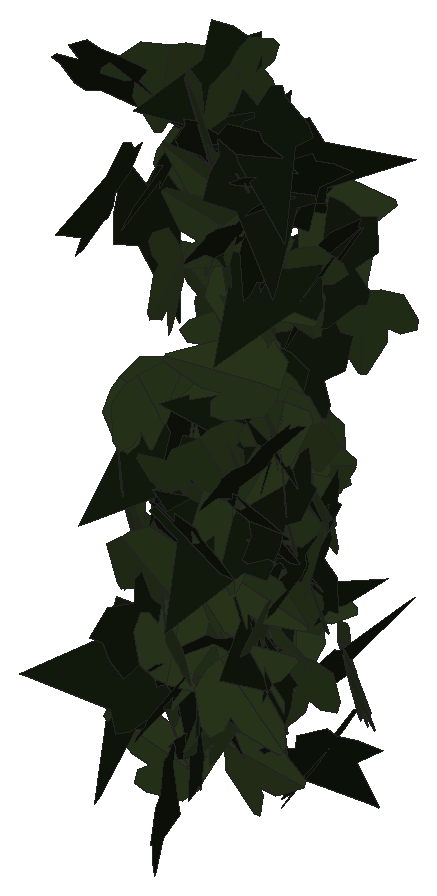
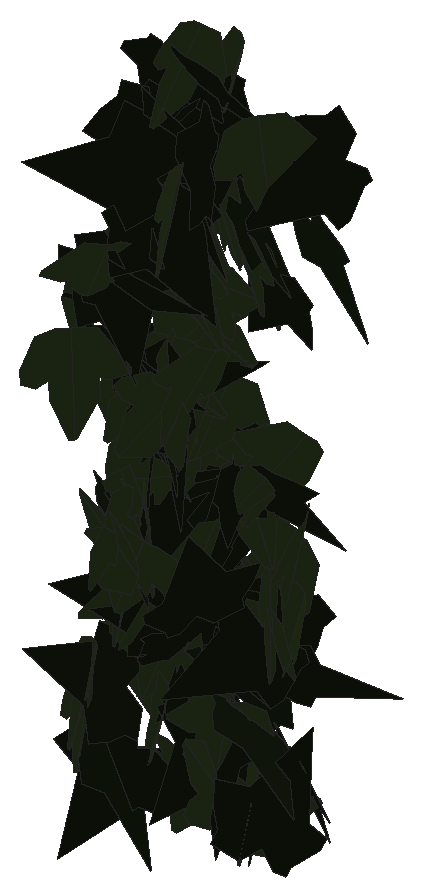
# SketchUp Ruby script. Lengths in inches.
U = 1.inch
M = Sketchup.active_model
def pt(a) = Geom::Point3d.new(a.map { |v| v * U })
def face(e, loops, mat)
  f = e.add_face(loops[0].map { |a| pt(a) })
  loops[1..].each { |l| e.add_face(l.map { |a| pt(a) }).erase! }
  f.material = f.back_material = mat if mat
  f
end
# faces: each face lists its corners as indices into pts; further lists are holes
def faces(e, pts, list, mat = nil) = list.each { |f| face(e, (f[0].is_a?(Array) ? f : [f]).map { |l| l.map { |i| pts[i] } }, mat) }
# xy, xz, yz: faces in a plane at the given z, y or x. An outline is a flat list of corners, or four numbers for a rectangle; further outlines are holes
def ring(l) = l.size == 4 ? [[l[0], l[1]], [l[2], l[1]], [l[2], l[3]], [l[0], l[3]]] : l.each_slice(2).to_a
def flat(e, list, mat, &to3) = list.each { |f| face(e, (f[0].is_a?(Array) ? f : [f]).map { |l| ring(l).map { |u, v| to3.(u, v) } }, mat) }
def xy(e, z, list, mat = nil) = flat(e, list, mat) { |x, y| [x, y, z] }
def xz(e, y, list, mat = nil) = flat(e, list, mat) { |x, z| [x, y, z] }
def yz(e, x, list, mat = nil) = flat(e, list, mat) { |y, z| [x, y, z] }
def lines(e, pts, list) = list.each { |a, b| e.add_line(pt(pts[a]), pt(pts[b])) }
# prism: a flat outline (further loops are holes) pulled along v
def prism(e, loops, v, mat = nil)
  f = face(e, loops, mat); d = Geom::Vector3d.new(v.map { |x| x * U })
  f.pushpull(f.normal.samedirection?(d) ? d.length : -d.length)
end
def box(e, o, s, mat = nil) = prism(e, [[o, [o[0] + s[0], o[1], o[2]], [o[0] + s[0], o[1] + s[1], o[2]], [o[0], o[1] + s[1], o[2]]]], [0, 0, s[2]], mat)
def at(x, y, z, deg = 0) = Geom::Transformation.translation(pt([x, y, z])) * Geom::Transformation.rotation(ORIGIN, Z_AXIS, deg.degrees)
def axes(o, x, y, z) = Geom::Transformation.new([*x, 0, *y, 0, *z, 0, *pt(o).to_a, 1])
def part(name) = M.definitions.add(name)
# library, detail: a bought-in or finely detailed component or shape, given as its bounding box
def library(name, o, s) = part(name).tap { |d| box(d.entities, o, s) }
def detail(e, o, s) = box(e.add_group.entities, o, s)
def put(e, d, t, mat = nil) = e.add_instance(d, t).tap { |i| i.material = mat if mat }
def group(e, t, mat = nil) = e.add_group.tap { |g| g.transformation = t; g.material = mat if mat }.entities
root = M.entities
M.materials.add("efeu1").color = [18, 25, 13]
M.materials.add("efeu2").color = [43, 57, 29]
c1 = part("ivyleaf_9")
p = [[1.54,2.16,1.25],[1.36,2.04,1.19],[-0.21,0.99,0.68],[-0.71,1.11,0.82],[-0.85,0.86,0.67],[-0.8,0.17,0.21],
  [-0.9,-0.01,0.1],[-0.67,-0.16,-0.02],[-0.08,-0.08,-0.05],[-0.03,-0.6,-0.4],[0.65,-0.88,-0.66],[0.83,-0.6,-0.49],
  [1.29,-0.42,-0.43],[1.8125,-0.07,-0.26],[1.21,0.44,0.15]]
faces(c1.entities,p,[[0,1,2,3,4,5,6,7,8,9,10,11,12,13,14]],"efeu1")
c2 = part("ivyleaf_10")
p = [[0,0.5,-0.03],[-0.0625,2.02,-0.43],[-0.19,2.01,-0.46],[-0.54,1.05,-0.29],[-0.52,0.625,-0.18],[-0.83,0.76,-0.28],
  [-1.16,0.64,-0.33],[-1.15,0.33,-0.24],[-0.77,-0.39,0.02],[-0.3,-0.51,0.16],[0.04,-0.48,0.23],[-0.02,2.01,-0.4375],
  [-0.06,2.01,-0.43],[0.04,-0.49,0.23],[0.67,-0.49,0.14],[1.38,0.36,-0.2],[1.375,0.51,-0.24],[0.81,0.65,-0.19],
  [0.62,0.59,-0.15],[0.6,1.09,-0.28],[0.5,1.23,-0.31]]
faces(c2.entities,p,[[0,1,2,3,4,5,6,7,8,9,10],[11,12,0,13,14,15,16,17,18,19,20]],"efeu2")
put(root,c1,axes([50.09,225.1875,214.06],[0.37177,-0.08571,0.32318],[-0.31461,0.07392,0.38152],[-0.11318,-0.48702,0.00103]))
put(root,c1,axes([49.87,224.07,222.45],[0.4848,0.06359,0.10454],[0.10369,0.01327,-0.48895],[-0.06496,0.49576,-0.00032]))
put(root,c2,axes([50.18,224.51,216.72],[-0.36902,0.33646,-0.02481],[0.00916,-0.02676,-0.4992],[-0.33725,-0.36889,0.01359]))
put(root,c1,axes([50.28,224.42,214.78],[-0.4013,0.06407,-0.29129],[0.2902,-0.02882,-0.40614],[-0.06883,-0.49504,-0.01405]))
put(root,c1,axes([50.54,223.71,221.2],[-0.31294,0.386,0.05546],[-0.02705,0.04945,-0.49681],[-0.38902,-0.31394,-0.01007]))
put(root,c2,axes([50.24,224.37,217.61],[-0.16912,0.46737,-0.05444],[0.00672,-0.05544,-0.49687],[-0.47048,-0.1688,0.01247]))
put(root,c1,axes([50.63,224.73,215.2],[-0.14528,0.43672,0.19536],[-0.19015,0.13464,-0.4424],[-0.43902,-0.20284,0.12697]))
put(root,c1,axes([50.5,225.86,217.19],[-0.28944,-0.24669,0.3246],[0.25134,0.20548,0.38027],[-0.32102,0.3833,0.00506]))
put(root,c2,axes([50.5,224.59,216.43],[-0.46152,0.18451,-0.05441],[-0.02286,-0.19302,-0.46067],[-0.191,-0.42273,0.1866]))
put(root,c2,axes([50.6,224.37,216.77],[0.08705,-0.42674,-0.24559],[-0.05203,0.24003,-0.43552],[0.48961,0.10138,-0.00261]))
put(root,c2,axes([50.85,224.59,213.82],[0.20562,0.14332,0.43264],[-0.37231,-0.22095,0.25014],[0.26288,-0.42502,0.01585]))
put(root,c1,axes([50.99,223.83,215.36],[-0.35853,0.0255,0.34757],[-0.34841,-0.03802,-0.3566],[0.00824,-0.4979,0.04503]))
put(root,c2,axes([50.72,224.45,222.61],[-0.33487,-0.36606,0.06215],[-0.03843,-0.04907,-0.4961],[0.36931,-0.33703,0.00473]))
put(root,c2,axes([50.78,224.49,214.39],[-0.32227,0.31708,0.21355],[-0.15272,0.14927,-0.4521],[-0.35046,-0.35662,0.00063]))
put(root,c2,axes([50.53,224.15,218.53],[0.15002,0.32465,0.34942],[0.10753,0.33385,-0.35635],[-0.46468,0.18207,0.03034]))
put(root,c1,axes([50.85,224.58,221.72],[-0.36486,0.27484,-0.20332],[0.15828,-0.12777,-0.45675],[-0.30302,-0.39767,0.00623]))
put(root,c1,axes([50.49,224.41,220.9],[-0.21631,-0.07779,-0.44403],[0.42341,0.13397,-0.22973],[0.15471,-0.4754,0.00792]))
put(root,c1,axes([50.45,224.5,216.25],[0.43193,0.14293,0.20739],[0.18332,0.10392,-0.45342],[-0.17272,0.46773,0.03737]))
put(root,c1,axes([50.95,224.33,218.04],[-0.48296,-0.11685,0.05568],[-0.05363,-0.0151,-0.49689],[0.1178,-0.48592,0.00205]))
put(root,c2,axes([50.66,224.18,218.52],[0.2277,0.3873,0.21943],[0.03568,0.2298,-0.44263],[-0.44371,0.21723,0.07701]))
put(root,c2,axes([50.84,224.61,221.35],[0.42787,-0.2583,0.01446],[0.01413,-0.00456,-0.49978],[0.25831,0.42809,0.00339]))
put(root,c1,axes([51.09,224.625,214.91],[0.288,0.05961,-0.40436],[-0.40809,0.01432,-0.28854],[-0.02282,0.49623,0.0569]))
put(root,c1,axes([50.96,224.62,218.37],[-0.13753,0.12973,-0.46288],[0.34145,-0.31253,-0.18904],[-0.33837,-0.3681,-0.00263]))
put(root,c2,axes([50.93,224.76,215.2],[0.43155,0.23257,0.09838],[0.04569,0.11966,-0.48332],[-0.24835,0.42614,0.08203]))
put(root,c1,axes([50.92,223.7,216.22],[0.00971,-0.04193,-0.49814],[-0.02923,0.49734,-0.04244],[0.49905,0.02994,0.00721]))
put(root,c2,axes([51.05,224.84,214.23],[0.15991,-0.41773,0.22346],[-0.08225,0.20778,0.44728],[-0.46654,-0.17981,-0.00227]))
put(root,c2,axes([50.92,223.7,216.875],[-0.38543,0.03402,-0.31668],[0.31527,-0.02992,-0.38692],[-0.04528,-0.49794,0.00162]))
put(root,c2,axes([50.89,224.6,215.1],[0.37806,-0.0655,0.3206],[0.31343,-0.06825,-0.38354],[0.09401,0.49097,-0.01055]))
put(root,c2,axes([51.42,223.92,217.7],[-0.40803,-0.06311,0.282],[-0.28032,-0.03213,-0.41278],[0.07022,-0.49496,-0.00916]))
put(root,c2,axes([51.1,225.02,219.78],[0.01707,0.44447,0.22838],[0.01799,0.22782,-0.44472],[-0.49938,0.0234,-0.00822]))
put(root,c1,axes([51.4,223.5,214.1],[0.04218,-0.02477,-0.4976],[-0.43677,0.23842,-0.04889],[0.2397,0.4388,-0.00152]))
put(root,c2,axes([51.41,225.15,222.0625],[-0.30758,0.2905,0.26647],[-0.182,0.19515,-0.42284],[-0.34968,-0.3571,-0.01431]))
put(root,c2,axes([51.52,223.49,216.25],[-0.33426,0.21349,0.30446],[-0.27075,0.14088,-0.39604],[-0.25489,-0.42962,0.02142]))
put(root,c1,axes([51.29,223.56,215.08],[-0.14693,0.44992,-0.16118],[-0.05192,0.1526,0.4733],[0.47509,0.15583,0.00188]))
put(root,c2,axes([51.46,223.59,220.66],[0.32655,-0.29998,-0.23103],[-0.15165,0.17592,-0.44278],[0.34693,0.35926,0.02391]))
put(root,c1,axes([51.35,224.3,214.62],[0.21407,0.38248,0.2406],[0.09858,0.22029,-0.4379],[-0.44097,0.23491,0.0189]))
put(root,c2,axes([51.74,224.03,220.18],[0.1499,-0.01815,0.47666],[-0.47396,0.05068,0.15098],[-0.0538,-0.49709,-0.00201]))
put(root,c1,axes([51.05,224.98,222.39],[0.13398,-0.03962,-0.48008],[0.47951,-0.03664,0.13684],[-0.04603,-0.49708,0.02818]))
put(root,c2,axes([51.71,223.92,221.29],[0.17798,-0.1305,-0.44866],[-0.28133,0.35339,-0.2144],[0.37306,0.32876,0.05237]))
put(root,c2,axes([51.51,224.47,217.17],[-0.09023,0.46214,0.16817],[-0.05152,0.16116,-0.4705],[-0.48909,-0.10224,0.01854]))
put(root,c2,axes([51.43,223.65,215.74],[0.4878,0.0947,-0.05557],[0.05366,0.01515,0.49688],[0.09579,-0.49072,0.00462]))
put(root,c1,axes([51.85,223.6,215],[-0.09695,0.08309,-0.48342],[-0.47846,0.09255,0.11186],[0.10807,0.48428,0.06157]))
put(root,c1,axes([51.87,224.13,216.15],[0.09094,0.12851,-0.47457],[-0.3863,-0.27988,-0.14981],[-0.30415,0.3939,0.04838]))
put(root,c1,axes([51.5,223.64,217.43],[0.45824,0.02672,-0.19825],[-0.19761,-0.01661,-0.45899],[-0.03112,0.49901,-0.00466]))
put(root,c1,axes([51.98,224.1,222.87],[-0.4259,0.16983,0.19942],[-0.19269,0.05472,-0.45812],[-0.17743,-0.46708,0.01884]))
put(root,c2,axes([51.45,225.3125,219.27],[-0.40736,0.07709,-0.27949],[0.26539,-0.09493,-0.41299],[-0.11674,-0.48481,0.03642]))
put(root,c1,axes([51.52,223.78,215.71],[0.34065,0.33509,0.14722],[0.09469,0.11358,-0.47763],[-0.35354,0.35329,0.01392]))
put(root,c2,axes([52.01,223.875,220.875],[0.02129,0.06543,0.49524],[-0.45944,0.19716,-0.0063],[-0.19611,-0.45481,0.06852]))
put(root,c1,axes([51.92,224.4375,216.87],[0.08918,0.02088,0.49154],[-0.47171,-0.13828,0.09146],[0.13976,-0.48004,-0.00497]))
put(root,c2,axes([51.61,224.42,214.89],[-0.018,-0.02441,0.49908],[0.18597,-0.46385,-0.01598],[0.46378,0.18506,0.02578]))
put(root,c1,axes([51.72,224.64,215.96],[-0.2736,-0.41776,0.02489],[-0.01899,-0.01732,-0.49934],[0.41807,-0.27418,-0.00639]))
put(root,c2,axes([51.58,224.01,216.29],[-0.43039,0.0132,-0.25415],[0.25235,-0.04257,-0.42955],[-0.03298,-0.49801,0.02998]))
put(root,c2,axes([51.79,224.21,218.61],[-0.24583,0.3806,0.21144],[-0.10415,0.18436,-0.45295],[-0.42275,-0.26675,-0.01136]))
put(root,c1,axes([52.16,224.32,215.76],[-0.29778,0.09709,0.38974],[-0.3736,0.11117,-0.31315],[-0.14747,-0.47772,0.00634]))
put(root,c2,axes([52.12,223.79,221.63],[-0.14741,0.04685,-0.47547],[-0.45802,0.12775,0.15459],[0.13596,0.48113,0.00525]))
put(root,c1,axes([52.01,224.39,218.72],[0.21192,0.00816,-0.4528],[-0.4527,0.01772,-0.21155],[0.01259,0.49962,0.01489]))
put(root,c2,axes([51.81,223.57,222.875],[-0.32496,0.37887,-0.02929],[0.01911,-0.0222,-0.49914],[-0.37952,-0.32552,-0.00005]))
put(root,c2,axes([51.64,225.46,217.375],[0.43734,0.12396,0.20825],[0.19811,0.0646,-0.45451],[-0.13959,0.48006,0.00739]))
put(root,c2,axes([52.12,223.91,221.14],[-0.29193,-0.11401,-0.38959],[-0.3378,-0.19788,0.31102],[-0.22511,0.4448,0.03851]))
put(root,c2,axes([51.84,225.78,217.76],[-0.03239,0.33209,-0.37238],[-0.05257,-0.37336,-0.32839],[-0.49617,0.01788,0.05911]))
put(root,c1,axes([51.95,224.05,217.52],[-0.39508,-0.3061,-0.01458],[0.01062,0.01011,-0.49979],[0.30627,-0.39522,-0.00149]))
put(root,c1,axes([52.19,223.93,215.46],[-0.03598,0.02806,0.49791],[-0.29441,0.40174,-0.04391],[-0.40253,-0.29634,-0.01238]))
put(root,c2,axes([51.51,224.79,214.14],[-0.01938,-0.04338,-0.49774],[0.4543,-0.20884,0.00052],[-0.20794,-0.45222,0.04751]))
put(root,c2,axes([52.05,224.0625,219.76],[0.33491,0.17112,-0.32947],[-0.30422,-0.12783,-0.37564],[-0.2128,0.45208,0.01849]))
put(root,c1,axes([52.09,224.62,221.26],[-0.02456,0.38752,-0.315],[-0.08003,-0.31436,-0.38049],[-0.49294,0.03173,0.07747]))
put(root,c2,axes([51.875,224.83,215.04],[-0.31168,0.38206,-0.08297],[0.03687,-0.07692,-0.49267],[-0.38922,-0.31323,0.01978]))
put(root,c2,axes([51.9,223.66,218.53],[-0.28854,-0.34588,-0.21706],[0.13072,0.17356,-0.45032],[0.38686,-0.31662,-0.00973]))
put(root,c2,axes([52.03,224.22,220.37],[0.44106,-0.13023,-0.19622],[-0.18907,0.05255,-0.45988],[0.14041,0.47987,-0.00289]))
put(root,c1,axes([52.27,224.3125,218.5],[-0.17782,0.05894,-0.46358],[-0.44074,0.14372,0.18733],[0.15533,0.47526,0.00084]))
put(root,c2,axes([52.23,224.67,217.33],[-0.18392,0.18107,0.42824],[-0.37638,0.21239,-0.25145],[-0.27297,-0.41485,0.05818]))
put(root,c1,axes([52.31,223.91,221.29],[-0.05238,0.00603,-0.49721],[-0.49714,-0.01112,0.05224],[-0.01043,0.49984,0.00716]))
put(root,c2,axes([51.91,224.1,215.49],[-0.13922,0.22191,0.42588],[0.17656,-0.38871,0.26026],[0.44659,0.22285,0.02987]))
put(root,c2,axes([51.94,224.06,217.72],[0.18128,0.46354,-0.04767],[-0.0095,-0.04746,-0.49765],[-0.46588,0.18133,-0.0084]))
put(root,c2,axes([51.92,223.9375,220.07],[-0.44965,0.08324,-0.20221],[0.19817,-0.04037,-0.45727],[-0.09245,-0.49137,0.00331]))
put(root,c2,axes([51.7,225.71,217.38],[0.16565,-0.1035,-0.46027],[0.38239,-0.25623,0.19524],[-0.27629,-0.41669,-0.00573]))
put(root,c1,axes([51.93,224.14,221.41],[-0.32683,0.03649,0.37663],[0.36104,-0.11892,0.32482],[0.11328,0.48428,0.05139]))
put(root,c2,axes([52.03,224.41,215.86],[-0.48259,0.06791,-0.11176],[0.1111,-0.01252,-0.48734],[-0.06899,-0.49521,-0.003]))
put(root,c2,axes([52.23,224.26,219.14],[-0.20338,0.24,0.38864],[-0.24977,0.29776,-0.31458],[-0.38243,-0.32209,-0.00123]))
put(root,c1,axes([52.4,224.47,218.74],[-0.17857,-0.07085,0.46162],[-0.42956,-0.16904,-0.19211],[0.18329,-0.46519,-0.0005]))
put(root,c1,axes([52.09,223.67,222.46],[0.40565,0.22791,-0.18304],[-0.1539,-0.09967,-0.46517],[-0.24852,0.43373,-0.01072]))
put(root,c2,axes([52.35,224.45,216.6],[-0.4223,-0.12058,0.23901],[-0.21781,-0.1048,-0.4377],[0.15565,-0.47379,0.03599]))
put(root,c2,axes([52.08,223.96,223.125],[-0.0792,-0.39506,-0.29607],[0.13872,0.26996,-0.39734],[0.4738,-0.14508,0.06685]))
put(root,c2,axes([52.43,224.28,219.04],[0.26292,0.0038,-0.42528],[-0.42523,-0.00606,-0.26294],[-0.00715,0.49995,0.00005]))
put(root,c2,axes([52.43,223.85,219.47],[0.08096,0.13233,0.47532],[-0.34022,-0.33388,0.1509],[0.35735,-0.34786,0.03598]))
put(root,c1,axes([52.33,224.05,220.61],[0.03721,0.14229,0.47788],[-0.04459,0.47824,-0.13892],[-0.49662,-0.03228,0.04828]))
put(root,c1,axes([52.35,224.45,217.81],[0.0559,-0.20852,0.451],[-0.04636,0.44967,0.21365],[-0.4947,-0.0657,0.03094]))
put(root,c2,axes([52.44,224.83,217.6],[-0.36754,0.15344,0.30228],[-0.2899,0.08884,-0.39758],[-0.17571,-0.46751,0.02366]))
put(root,c1,axes([52.62,224.72,219.2],[-0.27454,0.15888,0.38651],[-0.33228,0.19746,-0.31718],[-0.25342,-0.43101,-0.00284]))
put(root,c1,axes([52.37,223.6,221.51],[0.03508,0.4983,-0.02164],[-0.03296,-0.01933,-0.49854],[-0.49768,0.03641,0.03149]))
put(root,c1,axes([52.46,225.01,214.37],[-0.23105,0.4434,-0.00359],[-0.0005,-0.00431,-0.49998],[-0.44341,-0.23104,0.00243]))
put(root,c1,axes([52.61,224.75,216.93],[-0.106,0.00956,-0.48854],[-0.48014,-0.09487,0.10232],[-0.09074,0.49082,0.02929]))
put(root,c1,axes([52.02,223.98,217.73],[0.49829,-0.02069,-0.0357],[-0.03471,0.02373,-0.49823],[0.02231,0.49901,0.02221]))
put(root,c2,axes([52.21,224.45,216.11],[-0.06801,0.49202,-0.05739],[0.00093,-0.0578,-0.49665],[-0.49535,-0.06766,0.00695]))
put(root,c2,axes([52.63,224.52,217.59],[-0.18643,0.0822,-0.4566],[-0.41218,0.19654,0.20368],[0.21296,0.45234,-0.00552]))
put(root,c2,axes([52.29,224.24,216.39],[0.19593,-0.45831,0.03952],[0.01831,-0.03515,-0.49843],[0.45965,0.19676,0.00301]))
put(root,c2,axes([52.47,224.49,215.63],[-0.44696,-0.11978,0.18943],[-0.1755,-0.07578,-0.46201],[0.13939,-0.47949,0.0257]))
put(root,c1,axes([52.44,224.82,220.65],[-0.00036,0.48624,-0.1165],[0.00401,-0.11649,-0.48622],[-0.49998,-0.00128,-0.00381]))
put(root,c1,axes([52.59,224.62,217.15],[-0.17572,0.3595,0.2998],[-0.1185,0.27563,-0.39998],[-0.45286,-0.21162,-0.01166]))
put(root,c2,axes([52.05,224.02,220.58],[0.17363,0.2023,0.423],[0.25263,0.33964,-0.26613],[-0.39501,0.30614,0.01573]))
put(root,c1,axes([52.71,225.12,220.42],[-0.35707,0.04941,0.34649],[-0.34572,0.02734,-0.36018],[-0.05454,-0.4968,0.01464]))
put(root,c1,axes([52.03,224.38,218.71],[0.3589,-0.34484,0.04772],[0.03433,-0.03313,-0.49772],[0.34643,0.36054,-0.0001]))
put(root,c1,axes([52.21,224.88,214.35],[0.39868,0.30029,0.02961],[0.02613,0.01452,-0.49911],[-0.30061,0.39952,-0.00411]))
put(root,c1,axes([52.04,224.39,216.125],[0.17054,0.04342,0.46801],[0.42705,0.19364,-0.17358],[-0.19633,0.45893,0.02896]))
put(root,c2,axes([51.97,223.97,216.81],[0.1354,0.07233,0.47585],[0.44407,0.1719,-0.15248],[-0.18565,0.46392,-0.01769]))
put(root,c2,axes([52.68,224.41,218.75],[-0.23166,-0.09768,0.43219],[-0.38854,-0.18966,-0.25113],[0.213,-0.4522,0.01197]))
put(root,c1,axes([52.61,224.41,217.11],[-0.35055,0.35636,0.01089],[-0.00806,0.00735,-0.49988],[-0.35644,-0.35065,0.0006]))
put(root,c2,axes([52.46,224.68,216.7],[-0.3557,0.30344,0.1772],[-0.13969,0.10927,-0.46749],[-0.32244,-0.38208,0.00704]))
put(root,c1,axes([52.42,224.36,220.8],[-0.28442,-0.39806,0.10324],[-0.06162,-0.08285,-0.48922],[0.40658,-0.29101,-0.00193]))
put(root,c2,axes([52.3,224.68,216.34],[0.23061,0.44351,-0.01069],[-0.00498,-0.00946,-0.49989],[-0.44361,0.23067,0.00006]))
put(root,c2,axes([52.49,224.36,218.68],[0.20178,0.34304,-0.30267],[-0.18718,-0.23993,-0.39673],[-0.41743,0.27341,0.0316]))
put(root,c1,axes([52.28,224.28,215.96],[0.2413,-0.27931,-0.33728],[0.22842,-0.24828,0.36903],[-0.37363,-0.33218,0.00778]))
put(root,c2,axes([52.32,225.32,220.88],[0.16818,0.45234,0.13078],[0.05719,0.11822,-0.48245],[-0.46738,0.17724,-0.01198]))
put(root,c1,axes([52.77,223.89,217.82],[-0.14435,0.30045,0.37268],[-0.22321,0.30211,-0.33001],[-0.42348,-0.26165,0.04691]))
put(root,c2,axes([52.5625,225.58,219.72],[-0.42365,-0.25951,0.05636],[-0.05373,-0.02015,-0.4967],[0.26007,-0.4269,-0.01081]))
put(root,c2,axes([52.45,224.375,220.65],[-0.37541,-0.30376,-0.12959],[0.10598,0.07501,-0.48285],[0.31278,-0.39,0.00806]))
put(root,c1,axes([52.34,224.93,215.19],[-0.0371,0.47334,-0.15677],[-0.01462,0.1561,0.47478],[0.49841,0.03982,0.00226]))
put(root,c2,axes([52.63,225.26,215.3],[-0.34341,0.23796,0.27467],[-0.22164,0.16233,-0.41776],[-0.28799,-0.40869,-0.00601]))
put(root,c1,axes([52.64,224.97,220.54],[-0.23765,0.38679,-0.20956],[0.11585,-0.17475,-0.45392],[-0.42438,-0.26431,-0.00655]))
put(root,c1,axes([52.65,223.44,218.71],[-0.03487,0.49817,0.02478],[-0.00707,0.02434,-0.49936],[-0.49873,-0.03517,0.00535]))
put(root,c2,axes([52.31,223.59,215.84],[0.2278,0.35875,0.26345],[0.14191,0.22196,-0.42496],[-0.42186,0.26839,-0.00069]))
put(root,c2,axes([52.625,224.57,217.38],[0.3004,-0.32064,-0.23864],[-0.16223,0.17502,-0.43938],[0.3653,0.34141,0.00112]))
put(root,c1,axes([52.35,224.0625,222.03],[0.01389,-0.49632,-0.0589],[-0.00335,0.05883,-0.49652],[0.4998,0.01419,-0.0017]))
put(root,c1,axes([52.15,224.63,221.7],[0.24783,0.03225,0.43306],[0.42642,0.07623,-0.24971],[-0.08213,0.4931,0.01028]))
put(root,c1,axes([52.56,223.93,221.99],[0.24556,0.43448,-0.03043],[-0.01589,-0.02598,-0.49907],[-0.43526,0.24607,0.00105]))
put(root,c2,axes([52.62,225.21,215.52],[-0.35843,0.32325,0.13052],[-0.09186,0.09302,-0.48261],[-0.33629,-0.36994,-0.0073]))
put(root,c1,axes([52.37,223.95,222.77],[-0.26197,-0.15778,-0.39557],[0.34169,0.19935,-0.30579],[0.25421,-0.43054,0.00337]))
